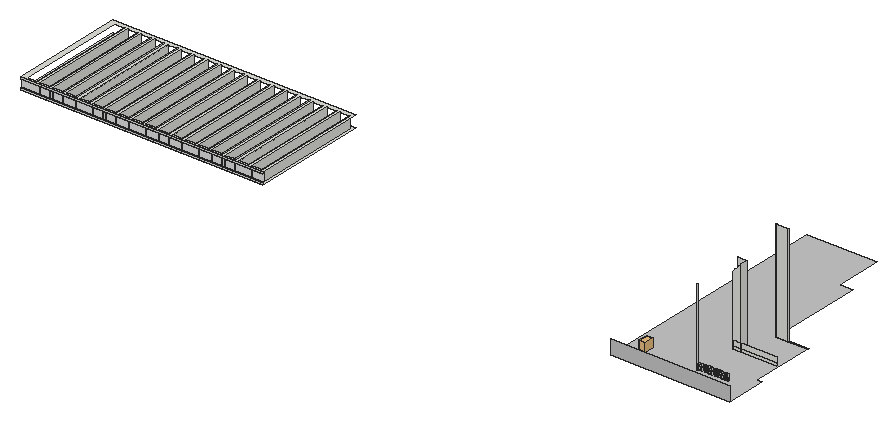
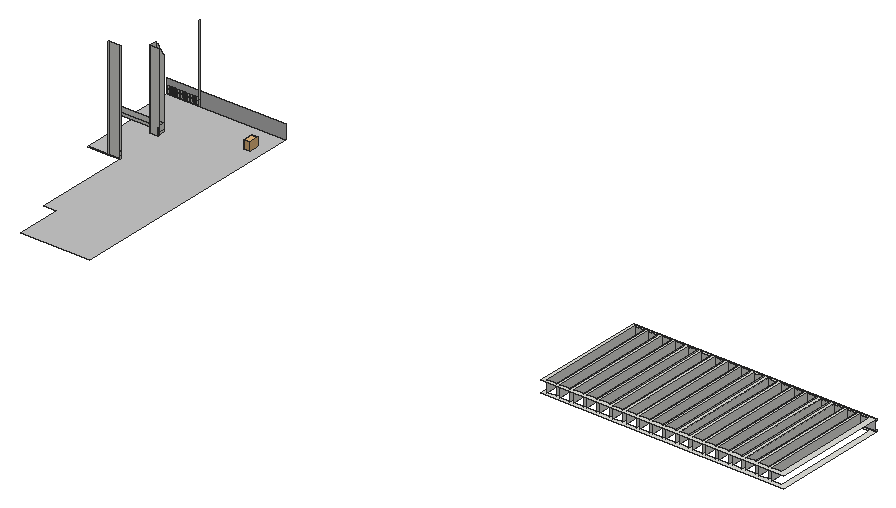
# SketchUp Ruby script. Lengths in inches.
U = 1.inch
M = Sketchup.active_model
def pt(a) = Geom::Point3d.new(a.map { |v| v * U })
def face(e, loops, mat)
  f = e.add_face(loops[0].map { |a| pt(a) })
  loops[1..].each { |l| e.add_face(l.map { |a| pt(a) }).erase! }
  f.material = f.back_material = mat if mat
  f
end
# faces: each face lists its corners as indices into pts; further lists are holes
def faces(e, pts, list, mat = nil) = list.each { |f| face(e, (f[0].is_a?(Array) ? f : [f]).map { |l| l.map { |i| pts[i] } }, mat) }
# xy, xz, yz: faces in a plane at the given z, y or x. An outline is a flat list of corners, or four numbers for a rectangle; further outlines are holes
def ring(l) = l.size == 4 ? [[l[0], l[1]], [l[2], l[1]], [l[2], l[3]], [l[0], l[3]]] : l.each_slice(2).to_a
def flat(e, list, mat, &to3) = list.each { |f| face(e, (f[0].is_a?(Array) ? f : [f]).map { |l| ring(l).map { |u, v| to3.(u, v) } }, mat) }
def xy(e, z, list, mat = nil) = flat(e, list, mat) { |x, y| [x, y, z] }
def xz(e, y, list, mat = nil) = flat(e, list, mat) { |x, z| [x, y, z] }
def yz(e, x, list, mat = nil) = flat(e, list, mat) { |y, z| [x, y, z] }
def lines(e, pts, list) = list.each { |a, b| e.add_line(pt(pts[a]), pt(pts[b])) }
# prism: a flat outline (further loops are holes) pulled along v
def prism(e, loops, v, mat = nil)
  f = face(e, loops, mat); d = Geom::Vector3d.new(v.map { |x| x * U })
  f.pushpull(f.normal.samedirection?(d) ? d.length : -d.length)
end
def box(e, o, s, mat = nil) = prism(e, [[o, [o[0] + s[0], o[1], o[2]], [o[0] + s[0], o[1] + s[1], o[2]], [o[0], o[1] + s[1], o[2]]]], [0, 0, s[2]], mat)
def at(x, y, z, deg = 0) = Geom::Transformation.translation(pt([x, y, z])) * Geom::Transformation.rotation(ORIGIN, Z_AXIS, deg.degrees)
def axes(o, x, y, z) = Geom::Transformation.new([*x, 0, *y, 0, *z, 0, *pt(o).to_a, 1])
def part(name) = M.definitions.add(name)
# library, detail: a bought-in or finely detailed component or shape, given as its bounding box
def library(name, o, s) = part(name).tap { |d| box(d.entities, o, s) }
def detail(e, o, s) = box(e.add_group.entities, o, s)
def put(e, d, t, mat = nil) = e.add_instance(d, t).tap { |i| i.material = mat if mat }
def group(e, t, mat = nil) = e.add_group.tap { |g| g.transformation = t; g.material = mat if mat }.entities
root = M.entities
M.materials.add("[Color M01]").color = [226, 226, 226]
M.materials.add("[Color M02]").color = [198, 198, 198]
c1 = library("Group\#13",[0,0,0],[3.54,3.54,3.9375])
xy(root,240.88,[[[1573.31,521.5625,1787.6875,623.84],[1776.28,523.31,1784.97,620.37],[1764.59,523.31,1773.28,620.37],[1752.91,523.31,1761.59,620.37],[1741.22,523.31,1749.91,620.37],[1729.53,523.31,1738.22,620.37],[1717.84,523.31,1726.53,620.37],[1706.16,523.31,1714.84,620.37],[1694.47,523.31,1703.16,620.37],[1682.78,523.31,1691.47,620.37],[1671.09,523.31,1679.78,620.37],[1659.41,523.31,1668.09,620.37],[1647.72,523.31,1656.41,620.37],[1636.03,523.31,1644.72,620.37],[1624.34,523.31,1633.03,620.37],[1612.66,523.31,1621.34,620.37],[1600.97,523.31,1609.66,620.37],[1589.28,523.31,1597.97,620.37],[1577.59,523.31,1586.28,620.37]]])
xy(root,242.34,[[1573.31,521.5625,1787.6875,522.8125]])
xy(root,249.61,[[1573.31,521.5625,1787.6875,522.8125]])
xy(root,251.0625,[[[1573.31,521.5625,1787.6875,623.84],[1776.28,523.31,1784.97,620.37],[1764.59,523.31,1773.28,620.37],[1752.91,523.31,1761.59,620.37],[1741.22,523.31,1749.91,620.37],[1729.53,523.31,1738.22,620.37],[1717.84,523.31,1726.53,620.37],[1706.16,523.31,1714.84,620.37],[1694.47,523.31,1703.16,620.37],[1682.78,523.31,1691.47,620.37],[1671.09,523.31,1679.78,620.37],[1659.41,523.31,1668.09,620.37],[1647.72,523.31,1656.41,620.37],[1636.03,523.31,1644.72,620.37],[1624.34,523.31,1633.03,620.37],[1612.66,523.31,1621.34,620.37],[1600.97,523.31,1609.66,620.37],[1589.28,523.31,1597.97,620.37],[1577.59,523.31,1586.28,620.37]],[2208.71,561.375,2219.52,562.32],[2219.52,561.375,2236.57,562.32]])
xy(root,251.0625,[[2135.95,469.875,2135.95,686.3125,2197.32,686.3125,2197.32,646.3125,2208.71,646.3125,2208.71,561.375,2236.57,561.375,2236.57,505.3125,2240.94,505.3125,2240.94,469.875]],"[Color M02]")
xy(root,257.0625,[[2202.51,521.5625,2208.71,528.48],[2208.71,521.5625,2209.43,528.48]])
xy(root,259.68,[[2205.66,480.14,2207.97,480.77],[2208.57,480.14,2210.89,480.77],[2211.49,480.14,2213.8,480.77],[2214.4,480.14,2216.71,480.77],[2217.31,480.14,2219.62,480.77],
  [2220.22,480.14,2222.53,480.77],[2223.13,480.14,2225.45,480.77],[2226.05,480.14,2228.36,480.77],[2228.96,480.14,2231.27,480.77]])
xy(root,262,[[2205.66,480.14,2207.97,480.77],[2208.57,480.14,2210.89,480.77],[2211.49,480.14,2213.8,480.77],[2214.4,480.14,2216.71,480.77],[2217.31,480.14,2219.62,480.77],
  [2220.22,480.14,2222.53,480.77],[2223.13,480.14,2225.45,480.77],[2226.05,480.14,2228.36,480.77],[2228.96,480.14,2231.27,480.77]])
xy(root,262.73,[[2205.69,480.14,2208,480.77],[2208.6,480.14,2210.92,480.77],[2211.52,480.14,2213.83,480.77],[2214.43,480.14,2216.74,480.77],[2217.34,480.14,2219.65,480.77],
  [2220.25,480.14,2222.5625,480.77],[2223.16,480.14,2225.48,480.77],[2226.08,480.14,2228.39,480.77],[2228.99,480.14,2231.3,480.77]])
xy(root,265.04,[[2205.69,480.14,2208,480.77],[2208.6,480.14,2210.92,480.77],[2211.52,480.14,2213.83,480.77],[2214.43,480.14,2216.74,480.77],[2217.34,480.14,2219.65,480.77],
  [2220.25,480.14,2222.5625,480.77],[2223.16,480.14,2225.48,480.77],[2226.08,480.14,2228.39,480.77],[2228.99,480.14,2231.3,480.77]])
xz(root,469.875,[[2135.95,251.0625,2240.94,263.89]],"[Color M02]")
xz(root,480.14,[[2203.9,258.95,2205.04,263.89],[2205.69,262.73,2208,263.89],[2208.6,262.73,2210.92,263.89],[2211.52,262.73,2213.83,263.89],[2214.43,262.73,2216.74,263.89],
  [2217.34,262.73,2219.65,263.89],[2220.25,262.73,2222.5625,263.89],[2223.16,262.73,2225.48,263.89],[2226.08,262.73,2228.39,263.89],[2228.99,262.73,2231.3,263.89]])
xz(root,480.77,[[2205.69,262.73,2208,263.89],[2208.6,262.73,2210.92,263.89],[2211.52,262.73,2213.83,263.89],[2214.43,262.73,2216.74,263.89],[2217.34,262.73,2219.65,263.89],
  [2220.25,262.73,2222.5625,263.89],[2223.16,262.73,2225.48,263.89],[2226.08,262.73,2228.39,263.89],[2228.99,262.73,2231.3,263.89]])
xz(root,521.5625,[[1573.31,240.88,1787.6875,242.34],[1573.31,249.61,1787.6875,251.0625],[2202.51,257.0625,2209.43,258.95],[2209.43,257.0625,2240.94,258.95],[2202.51,258.95,2209.43,263.89],
  [2209.43,258.95,2240.94,263.89],[2202.51,263.89,2209.43,263.89,2209.43,325.17,2208.49,324.17,2208.03,324.6,2207.16,323.67,2207.61,323.24,2205.19,320.67,2204.74,321.1,2203.86,320.17,2204.3125,319.74,2202.96,318.3,2202.51,317.82]])
xz(root,522.8125,[[1573.31,242.34,1787.6875,249.61]],"[Color M01]")
xz(root,523.31,[[1589.28,240.88,1597.97,251.0625],[1600.97,240.88,1609.66,251.0625],[1612.66,240.88,1621.34,251.0625],[1624.34,240.88,1633.03,251.0625],[1636.03,240.88,1644.72,251.0625],
  [1647.72,240.88,1656.41,251.0625],[1659.41,240.88,1668.09,251.0625],[1671.09,240.88,1679.78,251.0625],[1682.78,240.88,1691.47,251.0625],[1694.47,240.88,1703.16,251.0625],
  [1706.16,240.88,1714.84,251.0625],[1717.84,240.88,1726.53,251.0625],[1729.53,240.88,1738.22,251.0625],[1741.22,240.88,1749.91,251.0625],[1752.91,240.88,1761.59,251.0625],
  [1764.59,240.88,1773.28,251.0625],[1776.28,240.88,1784.97,251.0625]])
xz(root,528.48,[[2200.93,257.0625,2202.51,258.95],[2202.51,257.0625,2209.43,257.0625,2209.43,326.08,2200.93,326.08,2200.93,263.89,2202.51,263.89],[2200.93,258.95,2202.51,263.89]])
xz(root,561.375,[[2208.71,251.0625,2219.52,340.125]])
yz(root,1586.28,[[523.31,240.88,620.37,251.0625]])
yz(root,1589.28,[[523.31,240.88,620.37,251.0625]])
yz(root,1597.97,[[523.31,240.88,620.37,251.0625]])
yz(root,1600.97,[[523.31,240.88,620.37,251.0625]])
yz(root,1609.66,[[523.31,240.88,620.37,251.0625]])
yz(root,1612.66,[[523.31,240.88,620.37,251.0625]])
yz(root,1621.34,[[523.31,240.88,620.37,251.0625]])
yz(root,1624.34,[[523.31,240.88,620.37,251.0625]])
yz(root,1633.03,[[523.31,240.88,620.37,251.0625]])
yz(root,1636.03,[[523.31,240.88,620.37,251.0625]])
yz(root,1644.72,[[523.31,240.88,620.37,251.0625]])
yz(root,1647.72,[[523.31,240.88,620.37,251.0625]])
yz(root,1656.41,[[523.31,240.88,620.37,251.0625]])
yz(root,1659.41,[[523.31,240.88,620.37,251.0625]])
yz(root,1668.09,[[523.31,240.88,620.37,251.0625]])
yz(root,1671.09,[[523.31,240.88,620.37,251.0625]])
yz(root,1679.78,[[523.31,240.88,620.37,251.0625]])
yz(root,1682.78,[[523.31,240.88,620.37,251.0625]])
yz(root,1691.47,[[523.31,240.88,620.37,251.0625]])
yz(root,1694.47,[[523.31,240.88,620.37,251.0625]])
yz(root,1703.16,[[523.31,240.88,620.37,251.0625]])
yz(root,1706.16,[[523.31,240.88,620.37,251.0625]])
yz(root,1714.84,[[523.31,240.88,620.37,251.0625]])
yz(root,1717.84,[[523.31,240.88,620.37,251.0625]])
yz(root,1726.53,[[523.31,240.88,620.37,251.0625]])
yz(root,1729.53,[[523.31,240.88,620.37,251.0625]])
yz(root,1738.22,[[523.31,240.88,620.37,251.0625]])
yz(root,1741.22,[[523.31,240.88,620.37,251.0625]])
yz(root,1749.91,[[523.31,240.88,620.37,251.0625]])
yz(root,1752.91,[[523.31,240.88,620.37,251.0625]])
yz(root,1761.59,[[523.31,240.88,620.37,251.0625]])
yz(root,1764.59,[[523.31,240.88,620.37,251.0625]])
yz(root,1773.28,[[523.31,240.88,620.37,251.0625]])
yz(root,1776.28,[[523.31,240.88,620.37,251.0625]])
yz(root,1784.97,[[523.31,240.88,620.37,251.0625]])
yz(root,2202.51,[[521.5625,257.0625,528.48,258.95],[521.5625,258.95,528.48,263.89]])
yz(root,2203.9,[[480.14,258.95,480.77,263.89],[480.14,263.89,480.77,326.5]])
yz(root,2205.66,[[480.14,259.68,480.77,262]])
yz(root,2205.69,[[480.14,262.73,480.77,265.04]])
yz(root,2207.97,[[480.14,259.68,480.77,262]])
yz(root,2208,[[480.14,262.73,480.77,265.04]])
yz(root,2208.57,[[480.14,259.68,480.77,262]])
yz(root,2208.6,[[480.14,262.73,480.77,265.04]])
yz(root,2208.71,[[561.375,251.0625,562.32,253.4375],[561.375,253.4375,562.32,257.0625],[561.375,257.0625,562.32,340.125]])
yz(root,2209.43,[[521.5625,257.0625,528.48,326.08]])
yz(root,2210.89,[[480.14,259.68,480.77,262]])
yz(root,2210.92,[[480.14,262.73,480.77,265.04]])
yz(root,2211.49,[[480.14,259.68,480.77,262]])
yz(root,2211.52,[[480.14,262.73,480.77,265.04]])
yz(root,2213.8,[[480.14,259.68,480.77,262]])
yz(root,2213.83,[[480.14,262.73,480.77,265.04]])
yz(root,2214.4,[[480.14,259.68,480.77,262]])
yz(root,2214.43,[[480.14,262.73,480.77,265.04]])
yz(root,2216.71,[[480.14,259.68,480.77,262]])
yz(root,2216.74,[[480.14,262.73,480.77,265.04]])
yz(root,2217.31,[[480.14,259.68,480.77,262]])
yz(root,2217.34,[[480.14,262.73,480.77,265.04]])
yz(root,2219.52,[[561.375,251.0625,562.32,340.125]])
yz(root,2219.62,[[480.14,259.68,480.77,262]])
yz(root,2219.65,[[480.14,262.73,480.77,265.04]])
yz(root,2220.22,[[480.14,259.68,480.77,262]])
yz(root,2220.25,[[480.14,262.73,480.77,265.04]])
yz(root,2222.53,[[480.14,259.68,480.77,262]])
yz(root,2222.5625,[[480.14,262.73,480.77,265.04]])
yz(root,2223.13,[[480.14,259.68,480.77,262]])
yz(root,2223.16,[[480.14,262.73,480.77,265.04]])
yz(root,2225.45,[[480.14,259.68,480.77,262]])
yz(root,2225.48,[[480.14,262.73,480.77,265.04]])
yz(root,2226.05,[[480.14,259.68,480.77,262]])
yz(root,2226.08,[[480.14,262.73,480.77,265.04]])
yz(root,2228.36,[[480.14,259.68,480.77,262]])
yz(root,2228.39,[[480.14,262.73,480.77,265.04]])
yz(root,2228.96,[[480.14,259.68,480.77,262]])
yz(root,2228.99,[[480.14,262.73,480.77,265.04]])
yz(root,2231.27,[[480.14,259.68,480.77,262]])
yz(root,2231.3,[[480.14,262.73,480.77,265.04]])
yz(root,2231.87,[[480.14,259.68,480.77,262]])
p = [[2208.71,521.5625,251.0625],[2208.71,521.5625,257.0625],[2208.71,561.375,240.47],[2208.71,562.32,240.47],[2202.51,541.0625,251.0625],[2202.51,541.0625,253.4375],
  [2202.51,561.375,240.47]]
lines(root,p,[[0,1],[2,3],[4,5],[6,2]])
put(root,c1,axes([2151.5,488.625,258.17],[-1.5535,0,0],[0,2.39,0],[0,0,-3.63878]))
